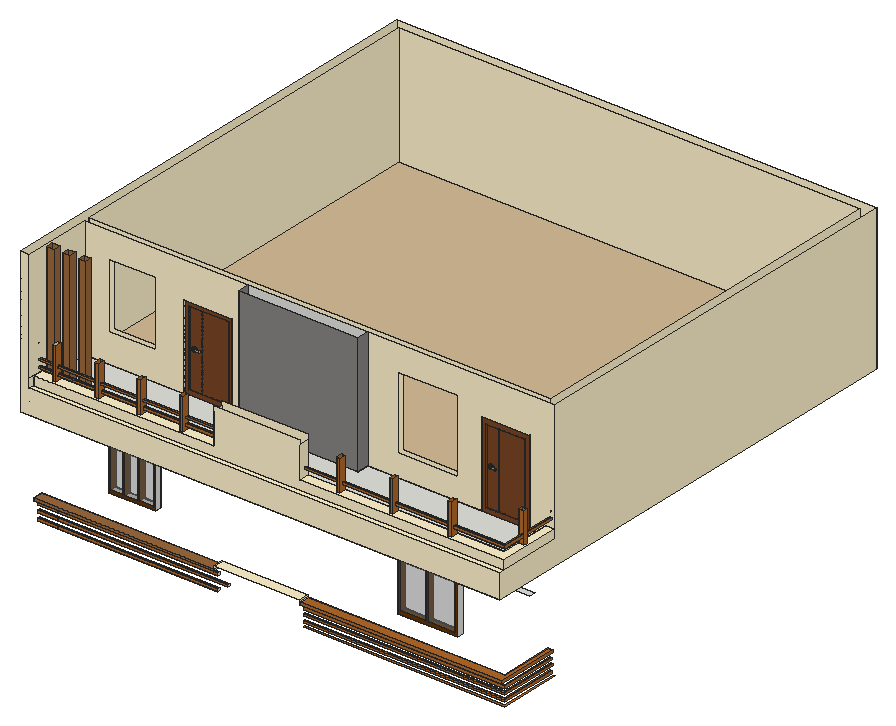
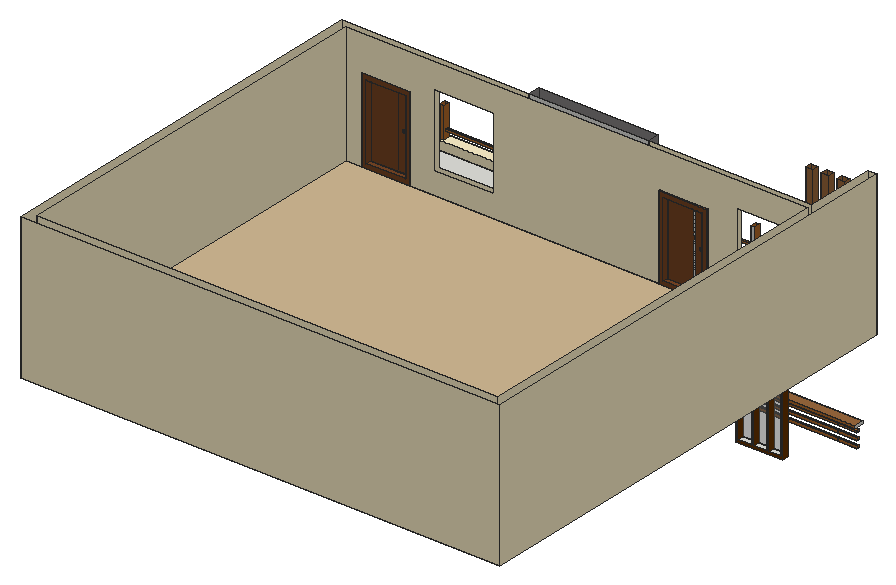
# SketchUp Ruby script. Lengths in inches.
U = 1.inch
M = Sketchup.active_model
def pt(a) = Geom::Point3d.new(a.map { |v| v * U })
def face(e, loops, mat)
  f = e.add_face(loops[0].map { |a| pt(a) })
  loops[1..].each { |l| e.add_face(l.map { |a| pt(a) }).erase! }
  f.material = f.back_material = mat if mat
  f
end
# faces: each face lists its corners as indices into pts; further lists are holes
def faces(e, pts, list, mat = nil) = list.each { |f| face(e, (f[0].is_a?(Array) ? f : [f]).map { |l| l.map { |i| pts[i] } }, mat) }
# xy, xz, yz: faces in a plane at the given z, y or x. An outline is a flat list of corners, or four numbers for a rectangle; further outlines are holes
def ring(l) = l.size == 4 ? [[l[0], l[1]], [l[2], l[1]], [l[2], l[3]], [l[0], l[3]]] : l.each_slice(2).to_a
def flat(e, list, mat, &to3) = list.each { |f| face(e, (f[0].is_a?(Array) ? f : [f]).map { |l| ring(l).map { |u, v| to3.(u, v) } }, mat) }
def xy(e, z, list, mat = nil) = flat(e, list, mat) { |x, y| [x, y, z] }
def xz(e, y, list, mat = nil) = flat(e, list, mat) { |x, z| [x, y, z] }
def yz(e, x, list, mat = nil) = flat(e, list, mat) { |y, z| [x, y, z] }
def lines(e, pts, list) = list.each { |a, b| e.add_line(pt(pts[a]), pt(pts[b])) }
# prism: a flat outline (further loops are holes) pulled along v
def prism(e, loops, v, mat = nil)
  f = face(e, loops, mat); d = Geom::Vector3d.new(v.map { |x| x * U })
  f.pushpull(f.normal.samedirection?(d) ? d.length : -d.length)
end
def box(e, o, s, mat = nil) = prism(e, [[o, [o[0] + s[0], o[1], o[2]], [o[0] + s[0], o[1] + s[1], o[2]], [o[0], o[1] + s[1], o[2]]]], [0, 0, s[2]], mat)
def at(x, y, z, deg = 0) = Geom::Transformation.translation(pt([x, y, z])) * Geom::Transformation.rotation(ORIGIN, Z_AXIS, deg.degrees)
def axes(o, x, y, z) = Geom::Transformation.new([*x, 0, *y, 0, *z, 0, *pt(o).to_a, 1])
def part(name) = M.definitions.add(name)
# library, detail: a bought-in or finely detailed component or shape, given as its bounding box
def library(name, o, s) = part(name).tap { |d| box(d.entities, o, s) }
def detail(e, o, s) = box(e.add_group.entities, o, s)
def put(e, d, t, mat = nil) = e.add_instance(d, t).tap { |i| i.material = mat if mat }
def group(e, t, mat = nil) = e.add_group.tap { |g| g.transformation = t; g.material = mat if mat }.entities
root = M.entities
M.materials.add("[Aluminum]").color = [179, 179, 179]
M.materials.add("[Brick Tumbled]").color = [135, 132, 132]
M.materials.add("[Color C08]").color = [102, 51, 0]
M.materials.add("[Color D01]").color = [255, 242, 204]
M.materials.add("[Formica Beige]").color = [211, 187, 149]
M.materials.add("[Translucent Glass Gray]").color = [128, 128, 128]
M.materials["[Translucent Glass Gray]"].alpha = 0.5
M.materials.add("[Wood Bamboo]").color = [177, 105, 43]
M.materials.add("[Wood Floor]").color = [155, 105, 61]
M.materials.add("[Wood Veneer 01]").color = [120, 70, 37]
c1 = part("Group\#4")
xy(c1.entities,0,[[0,0,52.875,9]],"[Color C08]")
xy(c1.entities,2.31,[[2.31,0,24.96,9],[26.98,0,50.56,9]],"[Color C08]")
xy(c1.entities,50.56,[[2.31,0,24.96,9],[26.98,0,50.56,9]],"[Color C08]")
xy(c1.entities,52.875,[[0,0,52.875,9]],"[Color C08]")
xz(c1.entities,0,[[[0,0,52.875,52.875],[26.98,2.31,50.56,50.56],[2.31,2.31,24.96,50.56]]],"[Color C08]")
xz(c1.entities,0,[[2.31,2.31,24.96,50.56],[26.98,2.31,50.56,50.56]],"[Translucent Glass Gray]")
xz(c1.entities,9,[[[0,0,52.875,52.875],[26.98,2.31,50.56,50.56],[2.31,2.31,24.96,50.56]]],"[Color C08]")
yz(c1.entities,0,[[0,0,9,52.875]],"[Color C08]")
yz(c1.entities,2.31,[[0,2.31,9,50.56]],"[Color C08]")
yz(c1.entities,24.96,[[0,2.31,9,50.56]],"[Color C08]")
yz(c1.entities,26.98,[[0,2.31,9,50.56]],"[Color C08]")
yz(c1.entities,50.56,[[0,2.31,9,50.56]],"[Color C08]")
yz(c1.entities,52.875,[[0,0,9,52.875]],"[Color C08]")
c2 = part("Group\#1")
xy(c2.entities,0,[[0,1.5625,48,2.9375],[0,2.9375,48,11.9375]],"[Wood Veneer 01]")
xy(c2.entities,4.26,[[4.26,1.5625,43.74,2.9375],[4.26,2.9375,43.74,11.9375]],"[Wood Veneer 01]")
xy(c2.entities,41.66,[[8.83,0,8.83,1.4375,9.58,1.4375,9.58,0.72,15.08,0.72,15.08,0]],"[Aluminum]")
xy(c2.entities,43.35,[[8.83,0,15.08,0,15.08,0.72,9.58,0.72,9.58,1.4375,8.83,1.4375]],"[Aluminum]")
xy(c2.entities,79.74,[[4.26,1.5625,16.16,2.9375],[16.16,1.5625,16.99,2.9375],[16.99,1.5625,43.74,2.9375],[4.26,2.9375,43.74,11.9375]],"[Wood Veneer 01]")
xy(c2.entities,84,[[0,1.5625,48,2.9375],[0,2.9375,48,11.9375]],"[Wood Veneer 01]")
xz(c2.entities,0,[[8.83,41.66,15.08,43.35]],"[Aluminum]")
xz(c2.entities,0.72,[[9.58,41.66,15.08,43.35]],"[Aluminum]")
xz(c2.entities,1.4375,[[[9.24,40.44,9.77,40.51,10.27,40.72,10.7,41.05,11.03,41.47,11.23,41.97,11.3,42.5,11.23,43.04,11.03,43.54,10.7,43.96,10.27,44.29,9.77,44.5,9.24,44.57,8.71,44.5,8.21,44.29,7.78,43.96,7.45,43.54,7.25,43.04,7.18,42.5,7.25,41.97,7.45,41.47,7.78,41.05,8.21,40.72,8.71,40.51],[8.83,41.66,9.58,43.35]]],"[Aluminum]")
xz(c2.entities,1.5625,[[[0,0,48,84],[4.26,4.26,43.74,79.74]]],"[Wood Veneer 01]")
xz(c2.entities,2.9375,[[[0,0,48,84],[4.26,4.26,43.74,79.74]],[16.16,4.26,16.99,79.74]])
xz(c2.entities,2.9375,[[[4.26,4.26,16.16,79.74],[9.24,40.44,8.71,40.51,8.21,40.72,7.78,41.05,7.45,41.47,7.25,41.97,7.18,42.5,7.25,43.04,7.45,43.54,7.78,43.96,8.21,44.29,8.71,44.5,9.24,44.57,9.77,44.5,10.27,44.29,10.7,43.96,11.03,43.54,11.23,43.04,11.3,42.5,11.23,41.97,11.03,41.47,10.7,41.05,10.27,40.72,9.77,40.51]],[16.99,4.26,43.74,79.74]],"[Wood Veneer 01]")
xz(c2.entities,11.9375,[[[0,0,48,84],[4.26,4.26,43.74,79.74]]],"[Wood Veneer 01]")
yz(c2.entities,0,[[1.5625,0,2.9375,84],[2.9375,0,11.9375,84]],"[Wood Veneer 01]")
yz(c2.entities,4.26,[[1.5625,4.26,2.9375,79.74],[2.9375,4.26,11.9375,79.74]],"[Wood Veneer 01]")
yz(c2.entities,8.83,[[0,41.66,1.4375,43.35]],"[Aluminum]")
yz(c2.entities,9.58,[[0.72,41.66,1.4375,43.35]],"[Aluminum]")
yz(c2.entities,15.08,[[0,41.66,0.72,43.35]],"[Aluminum]")
yz(c2.entities,43.74,[[1.5625,4.26,2.9375,79.74],[2.9375,4.26,11.9375,79.74]],"[Wood Veneer 01]")
yz(c2.entities,48,[[1.5625,0,2.9375,84],[2.9375,0,11.9375,84]],"[Wood Veneer 01]")
p = [[8.71,2.9375,40.51],[9.24,2.9375,40.44],[9.24,1.4375,40.44],[8.71,1.4375,40.51],[9.77,2.9375,40.51],[9.77,1.4375,40.51],
  [8.21,2.9375,40.72],[8.21,1.4375,40.72],[10.27,2.9375,40.72],[10.27,1.4375,40.72],[7.78,2.9375,41.05],[7.78,1.4375,41.05],
  [10.7,2.9375,41.05],[10.7,1.4375,41.05],[7.45,2.9375,41.47],[7.45,1.4375,41.47],[11.03,2.9375,41.47],[11.03,1.4375,41.47],
  [7.25,2.9375,41.97],[7.25,1.4375,41.97],[11.23,2.9375,41.97],[11.23,1.4375,41.97],[7.18,2.9375,42.5],[7.18,1.4375,42.5],
  [11.3,2.9375,42.5],[11.3,1.4375,42.5],[7.25,2.9375,43.04],[7.25,1.4375,43.04],[11.23,2.9375,43.04],[11.23,1.4375,43.04],
  [7.45,2.9375,43.54],[7.45,1.4375,43.54],[11.03,2.9375,43.54],[11.03,1.4375,43.54],[7.78,2.9375,43.96],[7.78,1.4375,43.96],
  [10.7,2.9375,43.96],[10.7,1.4375,43.96],[8.21,2.9375,44.29],[8.21,1.4375,44.29],[10.27,2.9375,44.29],[10.27,1.4375,44.29],
  [8.71,2.9375,44.5],[8.71,1.4375,44.5],[9.77,2.9375,44.5],[9.77,1.4375,44.5],[9.24,2.9375,44.57],[9.24,1.4375,44.57]]
faces(c2.entities,p,[[0,1,2,3],[1,4,5,2],[6,0,3,7],[4,8,9,5],[10,6,7,11],[8,12,13,9],[14,10,11,15],[12,16,17,13],
  [18,14,15,19],[16,20,21,17],[22,18,19,23],[20,24,25,21],[26,22,23,27],[24,28,29,25],[30,26,27,31],[28,32,33,29],
  [34,30,31,35],[32,36,37,33],[38,34,35,39],[36,40,41,37],[42,38,39,43],[40,44,45,41],[46,42,43,47],[44,46,47,45]],"[Aluminum]")
xy(root,162.24,[[274.98,145.89,477.01,145.89,477.01,207.71,475.1875,207.71,475.1875,148.02,274.98,148.02]],"[Wood Bamboo]")
xy(root,164.48,[[9,146.02,28.82,148.14]])
xy(root,164.48,[[28.82,146.02,189.63,148.14]],"[Wood Bamboo]")
xy(root,165.73,[[322.9,204.4,382.78,210.4]])
xy(root,166.24,[[274.98,145.89,274.98,148.02,475.1875,148.02,475.1875,204.4,477.01,204.4,477.01,145.89]],"[Wood Bamboo]")
xy(root,166.61,[[9,146.02,28.82,148.14],[28.82,146.02,189.63,148.14]],"[Wood Bamboo]")
xy(root,168.36,[[274.98,145.89,477.01,145.89,477.01,204.4,475.1875,204.4,475.1875,148.02,274.98,148.02]],"[Wood Bamboo]")
xy(root,171.67,[[9,146.02,28.82,148.14]])
xy(root,171.67,[[28.82,146.02,199.2,148.14]],"[Wood Bamboo]")
xy(root,172.43,[[274.98,145.89,274.98,148.02,475.1875,148.02,475.1875,205.64,477.01,205.64,477.01,145.89]],"[Wood Bamboo]")
xy(root,172.75,[[33.82,204.4,80.13,210.4]])
xy(root,173.8,[[9,146.02,28.82,148.14],[28.82,146.02,199.2,148.14]],"[Wood Bamboo]")
xy(root,174.55,[[274.98,145.89,477.01,145.89,477.01,205.64,475.1875,205.64,475.1875,148.02,274.98,148.02]],"[Wood Bamboo]")
xy(root,177.99,[[274.98,145.89,274.98,148.02,475.1875,148.02,475.1875,204.36,477.01,204.36,477.01,145.89]],"[Wood Bamboo]")
xy(root,178.55,[[9,146.02,28.82,148.14]])
xy(root,178.55,[[28.82,146.02,189.2,148.14]],"[Wood Bamboo]")
xy(root,180.49,[[274.98,145.89,477.01,145.89,477.01,204.36,475.1875,204.36,475.1875,148.02,274.98,148.02]],"[Wood Bamboo]")
xy(root,180.67,[[9,146.02,28.82,148.14],[28.82,146.02,189.2,148.14]],"[Wood Bamboo]")
xy(root,184,[[309.7,143.88,313.07,150.13]])
xy(root,184.18,[[[8.16,141.71,188.91,151.78],[68.13,143.88,71.51,150.13],[110.26,143.88,113.63,150.13]],[[274.98,141.71,274.98,151.78,472.375,151.78,472.375,205.65,477.34,205.65,477.34,141.71],[421.51,143.88,424.88,150.13]]],"[Wood Bamboo]")
xy(root,184.1875,[[472.3125,168.86,477.25,172.24]])
xy(root,184.4375,[[152.95,143.88,156.32,150.13]])
xy(root,184.5625,[[362.95,143.88,366.32,150.13]])
xy(root,185,[[25.45,143.88,28.82,150.13]])
xy(root,186.72,[[274.98,141.71,477.34,141.71,477.34,205.65,472.375,205.65,472.375,151.78,274.98,151.78]],"[Wood Bamboo]")
xy(root,186.72,[[8.16,141.71,188.91,151.78]],"[Wood Floor]")
xy(root,188.9375,[[188.91,140.9,274.98,151.78]],"[Color D01]")
xy(root,227.9375,[[108.75,204.4,156.75,210.4],[407.0625,204.4,455.0625,210.4]])
xy(root,238.56,[[33.82,204.4,80.13,210.4]])
xy(root,238.86,[[322.9,204.4,382.78,210.4]])
xy(root,263.9375,[[0,135.4,480,606.75]])
xy(root,263.9375,[[172.75,192.4,292.75,204.4]],"[Brick Tumbled]")
xy(root,263.9375,[[[0,135.4,9,135.4,9,204.4,480,204.4,480,606.75,0,606.75],[9,210.4,471,597.75]]],"[Color D01]")
xy(root,263.9375,[[11.75,154.17,19.6875,160.61],[27.8125,154.17,35,160.61],[43.5625,154.17,50.1875,160.61]],"[Wood Floor]")
xy(root,276.9375,[[9,151.78,9,204.4,108.75,204.4,108.75,210.4,156.75,210.4,156.75,204.4,172.75,204.4,172.75,192.4,292.75,192.4,292.75,204.4,407.0625,204.4,407.0625,210.4,455.0625,210.4,455.0625,204.4,471,204.4,471,151.78]])
xy(root,287.875,[[9,140.9,9,151.78,471,151.78,471,204.4,480,204.4,480,140.9],[[9,151.78,471,151.78,471,204.4,455.0625,204.4,455.0625,210.4,407.0625,210.4,407.0625,204.4,292.75,204.4,292.75,192.4,172.75,192.4,172.75,204.4,156.75,204.4,156.75,210.4,108.75,210.4,108.75,204.4,9,204.4],[11.75,154.17,19.6875,160.61],[27.8125,154.17,35,160.61],[43.5625,154.17,50.1875,160.61]],[172.75,192.4,292.75,204.4],[156.75,204.4,407.0625,210.4]])
xy(root,287.875,[[9,135.4,480,140.9]],"[Color D01]")
xy(root,287.875,[[9,210.4,471,597.75]],"[Formica Beige]")
xy(root,296.875,[[[9,140.9,188.91,151.78],[25.45,143.88,28.82,150.13],[68.13,143.88,71.51,150.13],[110.26,143.88,113.63,150.13],[152.95,143.88,156.32,150.13]],[[274.98,140.9,480,140.9,480,204.4,471,204.4,471,151.78,274.98,151.78],[309.7,143.88,313.07,150.13],[362.95,143.88,366.32,150.13],[421.51,143.88,424.88,150.13],[472.3125,168.86,477.25,172.24]]],"[Color D01]")
xy(root,301.08,[[9,146.22,28.82,148.34]])
xy(root,301.08,[[28.82,146.22,188.91,148.34]],"[Wood Bamboo]")
xy(root,303.21,[[9,146.22,28.82,148.34],[28.82,146.22,188.91,148.34]],"[Wood Bamboo]")
xy(root,304.05,[[274.98,145.89,274.98,148.02,475.1875,148.02,475.1875,207.71,477.01,207.71,477.01,145.89]],"[Wood Bamboo]")
xy(root,306.18,[[274.98,145.89,477.01,145.89,477.01,207.71,475.1875,207.71,475.1875,148.02,274.98,148.02]],"[Wood Bamboo]")
xy(root,308.42,[[9,146.02,28.82,148.14]])
xy(root,308.42,[[28.82,146.02,189.63,148.14]],"[Wood Bamboo]")
xz(root,135.4,[[0,263.9375,480,263.9375,480,287.875,9,287.875,9,407.875,0,407.875]],"[Color D01]")
xz(root,140.9,[[9,287.875,480,287.875,480,296.875,274.98,296.875,274.98,332.875,188.91,332.875,188.91,296.875,9,296.875]],"[Color D01]")
xz(root,141.71,[[274.98,184.18,477.34,186.72]],"[Wood Bamboo]")
xz(root,141.71,[[8.16,184.18,188.91,186.72]],"[Wood Floor]")
xz(root,143.88,[[25.45,296.875,28.82,328.9375],[68.13,296.875,71.51,328.12],[110.26,296.875,113.63,328.12],[152.95,296.875,156.32,328.375],[309.7,296.875,313.07,327.9375],
  [362.95,296.875,366.32,328.5],[421.51,296.875,424.88,328.12]],"[Wood Bamboo]")
xz(root,145.89,[[274.98,166.24,477.01,168.36],[274.98,172.43,477.01,174.55],[274.98,177.99,477.01,180.49],[274.98,304.05,477.01,306.18]],"[Wood Bamboo]")
xz(root,146.02,[[9,164.48,28.82,166.61],[28.82,164.48,189.63,166.61],[9,171.67,28.82,173.8],[28.82,171.67,199.2,173.8],[9,178.55,28.82,180.67],
  [28.82,178.55,189.2,180.67],[9,308.42,28.82,310.55],[28.82,308.42,189.63,310.55]],"[Wood Bamboo]")
xz(root,146.22,[[9,301.08,28.82,303.21],[28.82,301.08,188.91,303.21]],"[Wood Bamboo]")
xz(root,148.02,[[274.98,166.24,475.1875,168.36],[274.98,172.43,475.1875,174.55],[274.98,177.99,475.1875,180.49],[274.98,304.05,475.1875,306.18]],"[Wood Bamboo]")
xz(root,148.14,[[9,164.48,28.82,166.61],[28.82,164.48,189.63,166.61],[9,171.67,28.82,173.8],[28.82,171.67,199.2,173.8],[9,178.55,28.82,180.67],
  [28.82,178.55,189.2,180.67],[9,308.42,28.82,310.55],[28.82,308.42,189.63,310.55]],"[Wood Bamboo]")
xz(root,148.34,[[9,301.08,28.82,303.21],[28.82,301.08,188.91,303.21]],"[Wood Bamboo]")
xz(root,150.13,[[110.26,296.875,113.63,328.12],[152.95,296.875,156.32,328.375]])
xz(root,150.13,[[25.45,296.875,28.82,328.9375],[68.13,296.875,71.51,328.12],[309.7,296.875,313.07,327.9375],[362.95,296.875,366.32,328.5],[421.51,296.875,424.88,328.12]],"[Wood Bamboo]")
xz(root,151.78,[[9,276.9375,471,287.875]])
xz(root,151.78,[[9,287.875,9,296.875,188.91,296.875,188.91,332.875,274.98,332.875,274.98,296.875,471,296.875,471,287.875]],"[Color D01]")
xz(root,151.78,[[8.16,184.18,188.91,186.72],[274.98,184.18,472.375,186.72]],"[Wood Bamboo]")
xz(root,154.17,[[11.75,287.875,19.6875,407.875],[27.8125,287.875,35,407.875],[43.5625,287.875,50.1875,407.875]],"[Wood Floor]")
xz(root,160.61,[[11.75,287.875,19.6875,407.875],[27.8125,287.875,35,407.875],[43.5625,287.875,50.1875,407.875]],"[Wood Floor]")
xz(root,168.86,[[472.3125,296.875,477.25,328.125]],"[Wood Bamboo]")
xz(root,172.24,[[472.3125,296.875,477.25,328.125]],"[Wood Bamboo]")
xz(root,192.4,[[172.75,276.9375,292.75,287.875]])
xz(root,192.4,[[172.75,287.875,292.75,407.875]],"[Brick Tumbled]")
xz(root,204.36,[[475.1875,177.99,477.01,180.49]])
xz(root,204.4,[[9,276.9375,108.75,287.875],[156.75,276.9375,172.75,287.875],[292.75,276.9375,407.0625,287.875],[455.0625,276.9375,471,287.875],[172.75,287.875,292.75,407.875],
  [471,287.875,480,296.875]])
xz(root,204.4,[[[9,287.875,108.75,287.875,108.75,371.875,156.75,371.875,156.75,287.875,172.75,287.875,172.75,407.875,9,407.875],[33.82,316.68,80.13,382.5]],[[292.75,287.875,407.0625,287.875,407.0625,371.875,455.0625,371.875,455.0625,287.875,471,287.875,471,296.875,480,296.875,480,407.875,292.75,407.875],[322.9,309.67,382.78,382.8],[475.1875,310.18,477.01,312.3]]],"[Color D01]")
xz(root,205.64,[[475.1875,172.43,477.01,174.55]])
xz(root,205.65,[[472.375,184.18,477.34,186.72]])
xz(root,207.71,[[475.1875,304.05,477.01,306.18]])
xz(root,210.4,[[108.75,276.9375,156.75,287.875],[407.0625,276.9375,455.0625,287.875]])
xz(root,210.4,[[[9,287.875,9,407.875,471,407.875,471,287.875,455.0625,287.875,455.0625,371.875,407.0625,371.875,407.0625,287.875,156.75,287.875,156.75,371.875,108.75,371.875,108.75,287.875],[322.9,309.67,382.78,382.8],[33.82,316.68,80.13,382.5]]],"[Color D01]")
xz(root,597.75,[[9,287.875,471,407.875]],"[Color D01]")
xz(root,606.75,[[0,263.9375,480,407.875]],"[Color D01]")
yz(root,0,[[135.4,263.9375,606.75,407.875]],"[Color D01]")
yz(root,8.16,[[141.71,184.18,151.78,186.72]])
yz(root,9,[[151.78,276.9375,204.4,287.875],[140.9,287.875,151.78,296.875]])
yz(root,9,[[135.4,287.875,140.9,296.875],[[151.78,287.875,204.4,287.875,204.4,407.875,135.4,407.875,135.4,296.875,151.78,296.875],[146.02,322.48,148.14,324.61],[146.02,315.61,148.14,317.73],[146.02,308.42,148.14,310.55],[146.22,301.08,148.34,303.21]],[210.4,287.875,597.75,407.875]],"[Color D01]")
yz(root,11.75,[[154.17,287.875,160.61,407.875]],"[Wood Floor]")
yz(root,19.6875,[[154.17,287.875,160.61,407.875]],"[Wood Floor]")
yz(root,25.45,[[143.88,296.875,150.13,328.9375]])
yz(root,27.8125,[[154.17,287.875,160.61,407.875]],"[Wood Floor]")
yz(root,28.82,[[146.02,164.48,148.14,166.61],[146.02,171.67,148.14,173.8],[146.02,178.55,148.14,180.67],[146.22,301.08,148.34,303.21],[146.02,308.42,148.14,310.55]])
yz(root,28.82,[[[143.88,296.875,150.13,328.9375],[146.02,322.48,148.14,324.61],[146.02,315.61,148.14,317.73],[146.02,308.42,148.14,310.55],[146.22,301.08,148.34,303.21]]],"[Wood Bamboo]")
yz(root,33.82,[[204.4,172.75,210.4,238.56]])
yz(root,35,[[154.17,287.875,160.61,407.875]],"[Wood Floor]")
yz(root,43.5625,[[154.17,287.875,160.61,407.875]],"[Wood Floor]")
yz(root,50.1875,[[154.17,287.875,160.61,407.875]],"[Wood Floor]")
yz(root,68.13,[[143.88,296.875,150.13,328.12]],"[Wood Bamboo]")
yz(root,71.51,[[143.88,296.875,150.13,328.12]],"[Wood Bamboo]")
yz(root,80.13,[[204.4,172.75,210.4,238.56]])
yz(root,108.75,[[204.4,276.9375,210.4,287.875],[204.4,287.875,210.4,371.875]])
yz(root,110.26,[[143.88,296.875,150.13,328.12]],"[Wood Bamboo]")
yz(root,113.63,[[143.88,296.875,150.13,328.12]],"[Wood Bamboo]")
yz(root,152.95,[[143.88,296.875,150.13,328.375]],"[Wood Bamboo]")
yz(root,156.32,[[143.88,296.875,150.13,328.375]],"[Wood Bamboo]")
yz(root,156.75,[[204.4,276.9375,210.4,287.875],[204.4,287.875,210.4,371.875]])
yz(root,172.75,[[192.4,276.9375,204.4,287.875]])
yz(root,172.75,[[192.4,287.875,204.4,407.875]],"[Brick Tumbled]")
yz(root,188.91,[[141.71,184.18,151.78,186.72]])
yz(root,188.91,[[140.9,184.18,141.71,186.72],[140.9,186.72,151.78,188.9375],[[140.9,296.875,151.78,328.12],[146.22,301.08,148.34,303.21]]],"[Color D01]")
yz(root,189.2,[[146.02,178.55,148.14,180.67]])
yz(root,189.63,[[146.02,164.48,148.14,166.61],[146.02,308.42,148.14,310.55]])
yz(root,199.2,[[146.02,171.67,148.14,173.8]])
yz(root,274.98,[[141.71,184.18,151.78,186.72]])
yz(root,274.98,[[140.9,184.18,141.71,186.72],[140.9,186.72,151.78,188.9375],[[140.9,296.875,151.78,328.12],[145.89,321.93,148.02,324.43],[145.89,316.36,148.02,318.49],[145.89,310.18,148.02,312.3],[145.89,304.05,148.02,306.18]]],"[Color D01]")
yz(root,292.75,[[192.4,276.9375,204.4,287.875]])
yz(root,292.75,[[192.4,287.875,204.4,407.875]],"[Brick Tumbled]")
yz(root,309.7,[[143.88,296.875,150.13,327.9375]],"[Wood Bamboo]")
yz(root,313.07,[[143.88,296.875,150.13,327.9375]],"[Wood Bamboo]")
yz(root,322.9,[[204.4,165.73,210.4,238.86]])
yz(root,362.95,[[143.88,296.875,150.13,328.5]],"[Wood Bamboo]")
yz(root,366.32,[[143.88,296.875,150.13,328.5]],"[Wood Bamboo]")
yz(root,382.78,[[204.4,165.73,210.4,238.86]])
yz(root,407.0625,[[204.4,276.9375,210.4,287.875],[204.4,287.875,210.4,371.875]])
yz(root,421.51,[[143.88,296.875,150.13,328.12]],"[Wood Bamboo]")
yz(root,424.88,[[143.88,296.875,150.13,328.12]],"[Wood Bamboo]")
yz(root,455.0625,[[204.4,276.9375,210.4,287.875],[204.4,287.875,210.4,371.875]])
yz(root,471,[[151.78,276.9375,204.4,287.875]])
yz(root,471,[[151.78,287.875,204.4,296.875],[210.4,287.875,597.75,407.875]],"[Color D01]")
yz(root,472.3125,[[168.86,296.875,172.24,328.125]],"[Wood Bamboo]")
yz(root,472.375,[[151.78,184.18,205.65,186.72]],"[Wood Bamboo]")
yz(root,475.1875,[[148.02,166.24,204.4,168.36],[148.02,172.43,205.64,174.55],[148.02,177.99,204.36,180.49],[148.02,304.05,207.71,306.18]],"[Wood Bamboo]")
yz(root,477.01,[[145.89,166.24,204.4,168.36],[145.89,172.43,205.64,174.55],[145.89,177.99,204.36,180.49],[145.89,304.05,207.71,306.18]],"[Wood Bamboo]")
yz(root,477.25,[[168.86,296.875,172.24,328.125]],"[Wood Bamboo]")
yz(root,477.34,[[141.71,184.18,205.65,186.72]],"[Wood Bamboo]")
yz(root,480,[[135.4,263.9375,606.75,263.9375,606.75,407.875,204.4,407.875,204.4,287.875,135.4,287.875],[140.9,287.875,204.4,296.875]],"[Color D01]")
p = [[9,597.75,275.875],[9,597.75,287.875],[9,204.4,275.875],[9,204.4,276.9375],[471,204.4,275.875],[471,204.4,276.9375],
  [9,144.4,275.875],[9,135.4,275.875],[9,210.4,275.875],[9,210.4,287.875],[9,144.4,287.875],[471,597.75,275.875],
  [471,597.75,287.875],[471,210.4,275.875],[471,210.4,287.875]]
lines(root,p,[[0,1],[2,3],[4,5],[6,7],[8,9],[6,10],[11,12],[13,14]])
put(root,c1,axes([322.9,204.4,165.73],[1.13239,0,0],[0,0.62,0],[0,0,1.38298]))
g1 = group(root,at(33.75,204.4,172.75))
xy(g1,0,[[0,0,46.38,6.12]],"[Color C08]")
xy(g1,2.88,[[2.03,0,13.84,6.12],[15.61,0,28.92,6.12],[30.6875,0,44.35,6.12]])
xy(g1,62.93,[[2.03,0,13.84,6.12],[15.61,0,28.92,6.12],[30.6875,0,44.35,6.12]],"[Color C08]")
xy(g1,65.8125,[[0,0,46.38,6.12]],"[Color C08]")
xz(g1,0,[[[0,0,46.38,65.8125],[30.6875,2.88,44.35,62.93],[15.61,2.88,28.92,62.93],[2.03,2.88,13.84,62.93]]],"[Color C08]")
xz(g1,0,[[2.03,2.88,13.84,62.93],[15.61,2.88,28.92,62.93],[30.6875,2.88,44.35,62.93]],"[Translucent Glass Gray]")
xz(g1,6.12,[[[0,0,46.38,65.8125],[30.6875,2.88,44.35,62.93],[15.61,2.88,28.92,62.93],[2.03,2.88,13.84,62.93]]],"[Color C08]")
yz(g1,0,[[0,0,6.12,65.8125]],"[Color C08]")
yz(g1,2.03,[[0,2.88,6.12,62.93]],"[Color C08]")
yz(g1,13.84,[[0,2.88,6.12,62.93]],"[Color C08]")
yz(g1,15.61,[[0,2.88,6.12,62.93]],"[Color C08]")
yz(g1,28.92,[[0,2.88,6.12,62.93]],"[Color C08]")
yz(g1,30.6875,[[0,2.88,6.12,62.93]],"[Color C08]")
yz(g1,44.35,[[0,2.88,6.12,62.93]],"[Color C08]")
yz(g1,46.38,[[0,0,6.12,65.8125]],"[Color C08]")
g2 = group(root,at(407.0625,202.84,287.875))
xy(g2,0,[[0,1.02,48,1.91],[0,1.91,48,7.76]],"[Wood Veneer 01]")
xy(g2,4.26,[[4.26,1.02,43.74,1.91],[4.26,1.91,43.74,7.76]],"[Wood Veneer 01]")
xy(g2,41.66,[[8.83,0,8.83,0.93,9.58,0.93,9.58,0.47,15.08,0.47,15.08,0]],"[Aluminum]")
xy(g2,43.35,[[8.83,0,15.08,0,15.08,0.47,9.58,0.47,9.58,0.93,8.83,0.93]],"[Aluminum]")
xy(g2,79.74,[[4.26,1.02,16.16,1.91],[16.16,1.02,16.99,1.91],[16.99,1.02,43.74,1.91],[4.26,1.91,43.74,7.76]],"[Wood Veneer 01]")
xy(g2,84,[[0,1.02,48,1.91],[0,1.91,48,7.76]],"[Wood Veneer 01]")
xz(g2,0,[[8.83,41.66,15.08,43.35]],"[Aluminum]")
xz(g2,0.47,[[9.58,41.66,15.08,43.35]],"[Aluminum]")
xz(g2,0.93,[[[9.24,40.44,9.77,40.51,10.27,40.72,10.7,41.05,11.03,41.47,11.23,41.97,11.3,42.5,11.23,43.04,11.03,43.54,10.7,43.96,10.27,44.29,9.77,44.5,9.24,44.57,8.71,44.5,8.21,44.29,7.78,43.96,7.45,43.54,7.25,43.04,7.18,42.5,7.25,41.97,7.45,41.47,7.78,41.05,8.21,40.72,8.71,40.51],[8.83,41.66,9.58,43.35]]],"[Aluminum]")
xz(g2,1.02,[[[0,0,48,84],[4.26,4.26,43.74,79.74]]],"[Wood Veneer 01]")
xz(g2,1.91,[[[0,0,48,84],[4.26,4.26,43.74,79.74]],[16.16,4.26,16.99,79.74]])
xz(g2,1.91,[[[4.26,4.26,16.16,79.74],[9.24,40.44,8.71,40.51,8.21,40.72,7.78,41.05,7.45,41.47,7.25,41.97,7.18,42.5,7.25,43.04,7.45,43.54,7.78,43.96,8.21,44.29,8.71,44.5,9.24,44.57,9.77,44.5,10.27,44.29,10.7,43.96,11.03,43.54,11.23,43.04,11.3,42.5,11.23,41.97,11.03,41.47,10.7,41.05,10.27,40.72,9.77,40.51]],[16.99,4.26,43.74,79.74]],"[Wood Veneer 01]")
xz(g2,7.76,[[[0,0,48,84],[4.26,4.26,43.74,79.74]]],"[Wood Veneer 01]")
yz(g2,0,[[1.02,0,1.91,84],[1.91,0,7.76,84]],"[Wood Veneer 01]")
yz(g2,4.26,[[1.02,4.26,1.91,79.74],[1.91,4.26,7.76,79.74]],"[Wood Veneer 01]")
yz(g2,8.83,[[0,41.66,0.93,43.35]],"[Aluminum]")
yz(g2,9.58,[[0.47,41.66,0.93,43.35]],"[Aluminum]")
yz(g2,15.08,[[0,41.66,0.47,43.35]],"[Aluminum]")
yz(g2,43.74,[[1.02,4.26,1.91,79.74],[1.91,4.26,7.76,79.74]],"[Wood Veneer 01]")
yz(g2,48,[[1.02,0,1.91,84],[1.91,0,7.76,84]],"[Wood Veneer 01]")
p = [[8.71,1.91,40.51],[9.24,1.91,40.44],[9.24,0.93,40.44],[8.71,0.93,40.51],[9.77,1.91,40.51],[9.77,0.93,40.51],
  [8.21,1.91,40.72],[8.21,0.93,40.72],[10.27,1.91,40.72],[10.27,0.93,40.72],[7.78,1.91,41.05],[7.78,0.93,41.05],
  [10.7,1.91,41.05],[10.7,0.93,41.05],[7.45,1.91,41.47],[7.45,0.93,41.47],[11.03,1.91,41.47],[11.03,0.93,41.47],
  [7.25,1.91,41.97],[7.25,0.93,41.97],[11.23,1.91,41.97],[11.23,0.93,41.97],[7.18,1.91,42.5],[7.18,0.93,42.5],
  [11.3,1.91,42.5],[11.3,0.93,42.5],[7.25,1.91,43.04],[7.25,0.93,43.04],[11.23,1.91,43.04],[11.23,0.93,43.04],
  [7.45,1.91,43.54],[7.45,0.93,43.54],[11.03,1.91,43.54],[11.03,0.93,43.54],[7.78,1.91,43.96],[7.78,0.93,43.96],
  [10.7,1.91,43.96],[10.7,0.93,43.96],[8.21,1.91,44.29],[8.21,0.93,44.29],[10.27,1.91,44.29],[10.27,0.93,44.29],
  [8.71,1.91,44.5],[8.71,0.93,44.5],[9.77,1.91,44.5],[9.77,0.93,44.5],[9.24,1.91,44.57],[9.24,0.93,44.57]]
faces(g2,p,[[0,1,2,3],[1,4,5,2],[6,0,3,7],[4,8,9,5],[10,6,7,11],[8,12,13,9],[14,10,11,15],[12,16,17,13],
  [18,14,15,19],[16,20,21,17],[22,18,19,23],[20,24,25,21],[26,22,23,27],[24,28,29,25],[30,26,27,31],[28,32,33,29],
  [34,30,31,35],[32,36,37,33],[38,34,35,39],[36,40,41,37],[42,38,39,43],[40,44,45,41],[46,42,43,47],[44,46,47,45]],"[Aluminum]")
put(root,c2,axes([108.75,204.4,287.875],[1,0,0],[0,0.65,0],[0,0,1]))
